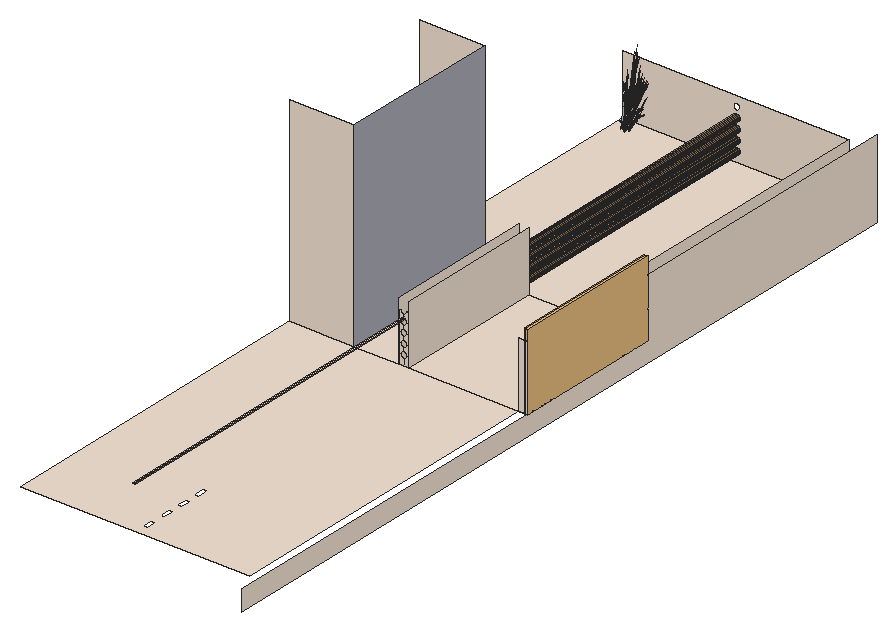
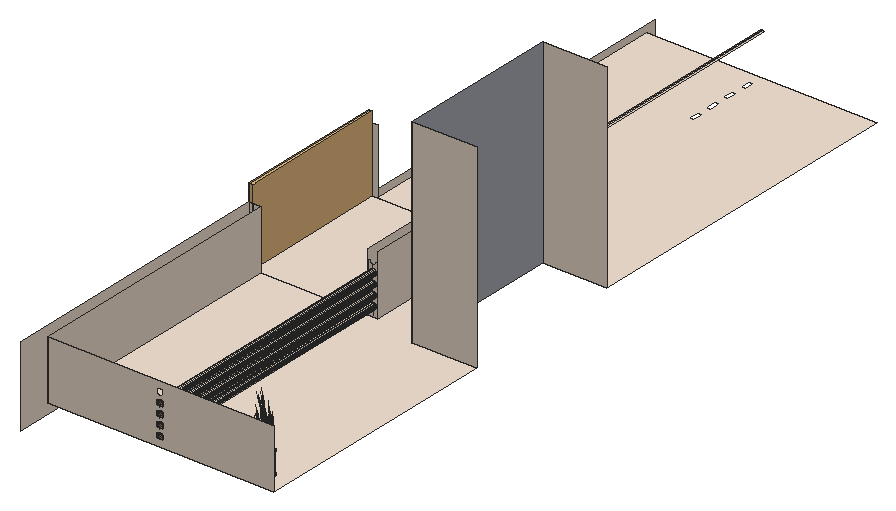
# SketchUp Ruby script. Lengths in inches.
U = 1.inch
M = Sketchup.active_model
def pt(a) = Geom::Point3d.new(a.map { |v| v * U })
def face(e, loops, mat)
  f = e.add_face(loops[0].map { |a| pt(a) })
  loops[1..].each { |l| e.add_face(l.map { |a| pt(a) }).erase! }
  f.material = f.back_material = mat if mat
  f
end
# faces: each face lists its corners as indices into pts; further lists are holes
def faces(e, pts, list, mat = nil) = list.each { |f| face(e, (f[0].is_a?(Array) ? f : [f]).map { |l| l.map { |i| pts[i] } }, mat) }
# xy, xz, yz: faces in a plane at the given z, y or x. An outline is a flat list of corners, or four numbers for a rectangle; further outlines are holes
def ring(l) = l.size == 4 ? [[l[0], l[1]], [l[2], l[1]], [l[2], l[3]], [l[0], l[3]]] : l.each_slice(2).to_a
def flat(e, list, mat, &to3) = list.each { |f| face(e, (f[0].is_a?(Array) ? f : [f]).map { |l| ring(l).map { |u, v| to3.(u, v) } }, mat) }
def xy(e, z, list, mat = nil) = flat(e, list, mat) { |x, y| [x, y, z] }
def xz(e, y, list, mat = nil) = flat(e, list, mat) { |x, z| [x, y, z] }
def yz(e, x, list, mat = nil) = flat(e, list, mat) { |y, z| [x, y, z] }
def lines(e, pts, list) = list.each { |a, b| e.add_line(pt(pts[a]), pt(pts[b])) }
# prism: a flat outline (further loops are holes) pulled along v
def prism(e, loops, v, mat = nil)
  f = face(e, loops, mat); d = Geom::Vector3d.new(v.map { |x| x * U })
  f.pushpull(f.normal.samedirection?(d) ? d.length : -d.length)
end
def box(e, o, s, mat = nil) = prism(e, [[o, [o[0] + s[0], o[1], o[2]], [o[0] + s[0], o[1] + s[1], o[2]], [o[0], o[1] + s[1], o[2]]]], [0, 0, s[2]], mat)
def at(x, y, z, deg = 0) = Geom::Transformation.translation(pt([x, y, z])) * Geom::Transformation.rotation(ORIGIN, Z_AXIS, deg.degrees)
def axes(o, x, y, z) = Geom::Transformation.new([*x, 0, *y, 0, *z, 0, *pt(o).to_a, 1])
def part(name) = M.definitions.add(name)
# library, detail: a bought-in or finely detailed component or shape, given as its bounding box
def library(name, o, s) = part(name).tap { |d| box(d.entities, o, s) }
def detail(e, o, s) = box(e.add_group.entities, o, s)
def put(e, d, t, mat = nil) = e.add_instance(d, t).tap { |i| i.material = mat if mat }
def group(e, t, mat = nil) = e.add_group.tap { |g| g.transformation = t; g.material = mat if mat }.entities
root = M.entities
M.materials.add("C01_Vanilla_Cream").color = [244, 228, 212]
M.materials.add("LightPink_Translucent").color = [144, 107, 117]
M.materials["LightPink_Translucent"].alpha = 0.75
M.materials.add("Marble_20_1K").color = [172, 173, 182]
M.materials.add("Wood_Floor_01_1K").color = [146, 111, 76]
c1 = part("blade")
p = [[2.15,0.21,22],[0,0.17,0],[0.09,0.45,0],[2.18,0.31,22],[2.29,0.31,22],[0.38,0.45,0],
  [2.48,0.24,33],[2.49,0.24,33],[2.48,0.22,33]]
faces(c1.entities,p,[[0,1,2,3],[4,5,2,3],[6,3,4,7],[8,0,3,6]])
c2 = part("seeds")
p = [[0.3,-0.1,1.38],[-0.01,-0.03,1.59],[-0.01,-0.03,0.03],[0.14,-0.07,-0.07],[0.29,-0.03,3],[0.15,0.01,3.11]]
faces(c2.entities,p,[[0,1,2,3],[1,0,4,5]],"LightPink_Translucent")
c3 = part("blade with seeds")
put(c3.entities,c1,at(0,0,0))
put(c3.entities,c2,axes([2.4,0.25,30.99],[1.5799,-0.05474,1.17369],[-0.12525,1.92788,0.29478],[-0.07173,-0.02425,1.56792]))
c4 = library("Modern+Gate+1",[0,0,0],[118.11,1.97,78.74])
xy(root,12,[[[288,12,426.72,216],[357,44.28,360,50.74],[357,18.46,360,24.91],[357,31.37,360,37.83],[357,57.2,360,63.65]],[326.85,216,354,216,354,306.76,424.7,306.76,424.7,468,288,468,288,314.71,326.85,314.71],[354,216,360,306.76],[360,216,432,306.76]],"C01_Vanilla_Cream")
xz(root,216,[[288,12,326.85,132],[354,12,357,12,357,16,356.48,16.07,356,16.27,355.59,16.59,355.27,17,355.07,17.48,355,18,354,18],[357,12,360,12,360,18,359,18,358.93,17.48,358.73,17,358.41,16.59,358,16.27,357.52,16.07,357,16],[426.72,12,432,51.56],[354,18,355,18,355.07,18.52,355.27,19,355.59,19.41,356,19.73,356.48,19.93,357,20,357,22,356.48,22.07,356,22.27,355.59,22.59,355.27,23,355.07,23.48,355,24,354,24],
  [359,18,360,18,360,24,359,24,358.93,23.48,358.73,23,358.41,22.59,358,22.27,357.52,22.07,357,22,357,20,357.52,19.93,358,19.73,358.41,19.41,358.73,19,358.93,18.52],[354,24,355,24,355.07,24.52,355.27,25,355.59,25.41,356,25.73,356.48,25.93,357,26,357,28,356.48,28.07,356,28.27,355.59,28.59,355.27,29,355.07,29.48,355,30,354,30],[359,24,360,24,360,30,359,30,358.93,29.48,358.73,29,358.41,28.59,358,28.27,357.52,28.07,357,28,357,26,357.52,25.93,358,25.73,358.41,25.41,358.73,25,358.93,24.52],[354,30,355,30,355.07,30.52,355.27,31,355.59,31.41,356,31.73,356.48,31.93,357,32,357,34,356.48,34.07,356,34.27,355.59,34.59,355.27,35,355.07,35.48,355,36,354,36],[359,30,360,30,360,36,359,36,358.93,35.48,358.73,35,358.41,34.59,358,34.27,357.52,34.07,357,34,357,32,357.52,31.93,358,31.73,358.41,31.41,358.73,31,358.93,30.52],
  [354,36,355,36,355.07,36.52,355.27,37,355.59,37.41,356,37.73,356.48,37.93,357,38,357,40,356.48,40.07,356,40.27,355.59,40.59,355.27,41,355.07,41.48,355,42,354,42],[359,36,360,36,360,42,359,42,358.93,41.48,358.73,41,358.41,40.59,358,40.27,357.52,40.07,357,40,357,38,357.52,37.93,358,37.73,358.41,37.41,358.73,37,358.93,36.52]],"C01_Vanilla_Cream")
xz(root,306.76,[[354,12,354,18,355,18,355.07,17.48,355.27,17,355.59,16.59,356,16.27,356.48,16.07,357,16,357,12],[357,12,357,16,357.52,16.07,358,16.27,358.41,16.59,358.73,17,358.93,17.48,359,18,360,18,360,12],[424.7,12,432,48],[354,18,354,24,355,24,355.07,23.48,355.27,23,355.59,22.59,356,22.27,356.48,22.07,357,22,357,20,356.48,19.93,356,19.73,355.59,19.41,355.27,19,355.07,18.52,355,18],[359,18,358.93,18.52,358.73,19,358.41,19.41,358,19.73,357.52,19.93,357,20,357,22,357.52,22.07,358,22.27,358.41,22.59,358.73,23,358.93,23.48,359,24,360,24,360,18],
  [354,24,354,30,355,30,355.07,29.48,355.27,29,355.59,28.59,356,28.27,356.48,28.07,357,28,357,26,356.48,25.93,356,25.73,355.59,25.41,355.27,25,355.07,24.52,355,24],[359,24,358.93,24.52,358.73,25,358.41,25.41,358,25.73,357.52,25.93,357,26,357,28,357.52,28.07,358,28.27,358.41,28.59,358.73,29,358.93,29.48,359,30,360,30,360,24],[354,30,354,36,355,36,355.07,35.48,355.27,35,355.59,34.59,356,34.27,356.48,34.07,357,34,357,32,356.48,31.93,356,31.73,355.59,31.41,355.27,31,355.07,30.52,355,30],[359,30,358.93,30.52,358.73,31,358.41,31.41,358,31.73,357.52,31.93,357,32,357,34,357.52,34.07,358,34.27,358.41,34.59,358.73,35,358.93,35.48,359,36,360,36,360,30],[354,36,354,42,355,42,355.07,41.48,355.27,41,355.59,40.59,356,40.27,356.48,40.07,357,40,357,38,356.48,37.93,356,37.73,355.59,37.41,355.27,37,355.07,36.52,355,36],
  [359,36,358.93,36.52,358.73,37,358.41,37.41,358,37.73,357.52,37.93,357,38,357,40,357.52,40.07,358,40.27,358.41,40.59,358.73,41,358.93,41.48,359,42,360,42,360,36]],"C01_Vanilla_Cream")
xz(root,314.71,[[288,12,326.85,132]],"C01_Vanilla_Cream")
xz(root,468,[[[288,12,424.7,48],[357,40,356.48,40.07,356,40.27,355.59,40.59,355.27,41,355.07,41.48,355,42,355.07,42.52,355.27,43,355.59,43.41,356,43.73,356.48,43.93,357,44,357.52,43.93,358,43.73,358.41,43.41,358.73,43,358.93,42.52,359,42,358.93,41.48,358.73,41,358.41,40.59,358,40.27,357.52,40.07],[357,34,356.48,34.07,356,34.27,355.59,34.59,355.27,35,355.07,35.48,355,36,355.07,36.52,355.27,37,355.59,37.41,356,37.73,356.48,37.93,357,38,357.52,37.93,358,37.73,358.41,37.41,358.73,37,358.93,36.52,359,36,358.93,35.48,358.73,35,358.41,34.59,358,34.27,357.52,34.07],[357,28,356.48,28.07,356,28.27,355.59,28.59,355.27,29,355.07,29.48,355,30,355.07,30.52,355.27,31,355.59,31.41,356,31.73,356.48,31.93,357,32,357.52,31.93,358,31.73,358.41,31.41,358.73,31,358.93,30.52,359,30,358.93,29.48,358.73,29,358.41,28.59,358,28.27,357.52,28.07],[357,22,356.48,22.07,356,22.27,355.59,22.59,355.27,23,355.07,23.48,355,24,355.07,24.52,355.27,25,355.59,25.41,356,25.73,356.48,25.93,357,26,357.52,25.93,358,25.73,358.41,25.41,358.73,25,358.93,24.52,359,24,358.93,23.48,358.73,23,358.41,22.59,358,22.27,357.52,22.07],[357,16,356.48,16.07,356,16.27,355.59,16.59,355.27,17,355.07,17.48,355,18,355.07,18.52,355.27,19,355.59,19.41,356,19.73,356.48,19.93,357,20,357.52,19.93,358,19.73,358.41,19.41,358.73,19,358.93,18.52,359,18,358.93,17.48,358.73,17,358.41,16.59,358,16.27,357.52,16.07]]],"C01_Vanilla_Cream")
yz(root,326.85,[[216,12,314.71,132]],"Marble_20_1K")
yz(root,354,[[216,12,306.76,48]],"C01_Vanilla_Cream")
yz(root,360,[[216,12,306.76,48]],"C01_Vanilla_Cream")
yz(root,424.7,[[306.76,12,468,48]],"C01_Vanilla_Cream")
yz(root,432,[[0,0,480,0,480,48,306.76,48,306.76,12,0,12]],"C01_Vanilla_Cream")
p = [[357,306.76,16],[356.48,306.76,16.07],[356.48,468,16.07],[357,468,16],[357.52,306.76,16.07],[357.52,468,16.07],
  [356,306.76,16.27],[356,468,16.27],[358,306.76,16.27],[358,468,16.27],[355.59,306.76,16.59],[355.59,468,16.59],
  [358.41,306.76,16.59],[358.41,468,16.59],[355.27,306.76,17],[355.27,468,17],[358.73,306.76,17],[358.73,468,17],
  [355.07,306.76,17.48],[355.07,468,17.48],[358.93,306.76,17.48],[358.93,468,17.48],[355,306.76,18],[355,468,18],
  [359,306.76,18],[359,468,18],[355.07,306.76,18.52],[355.07,468,18.52],[358.93,306.76,18.52],[358.93,468,18.52],
  [355.27,306.76,19],[355.27,468,19],[358.73,306.76,19],[358.73,468,19],[355.59,306.76,19.41],[355.59,468,19.41],
  [358.41,306.76,19.41],[358.41,468,19.41],[356,306.76,19.73],[356,468,19.73],[358,306.76,19.73],[358,468,19.73],
  [356.48,306.76,19.93],[356.48,468,19.93],[357.52,306.76,19.93],[357.52,468,19.93],[357,306.76,20],[357,468,20],
  [357,306.76,22],[356.48,306.76,22.07],[356.48,468,22.07],[357,468,22],[357.52,306.76,22.07],[357.52,468,22.07],
  [356,306.76,22.27],[356,468,22.27],[358,306.76,22.27],[358,468,22.27],[355.59,306.76,22.59],[355.59,468,22.59],
  [358.41,306.76,22.59],[358.41,468,22.59],[355.27,306.76,23],[355.27,468,23],[358.73,306.76,23],[358.73,468,23],
  [355.07,306.76,23.48],[355.07,468,23.48],[358.93,306.76,23.48],[358.93,468,23.48],[355,306.76,24],[355,468,24],
  [359,306.76,24],[359,468,24],[355.07,306.76,24.52],[355.07,468,24.52],[358.93,306.76,24.52],[358.93,468,24.52],
  [355.27,306.76,25],[355.27,468,25],[358.73,306.76,25],[358.73,468,25],[355.59,306.76,25.41],[355.59,468,25.41],
  [358.41,306.76,25.41],[358.41,468,25.41],[356,306.76,25.73],[356,468,25.73],[358,306.76,25.73],[358,468,25.73],
  [356.48,306.76,25.93],[356.48,468,25.93],[357.52,306.76,25.93],[357.52,468,25.93],[357,306.76,26],[357,468,26],
  [357,306.76,28],[356.48,306.76,28.07],[356.48,468,28.07],[357,468,28],[357.52,306.76,28.07],[357.52,468,28.07],
  [356,306.76,28.27],[356,468,28.27],[358,306.76,28.27],[358,468,28.27],[355.59,306.76,28.59],[355.59,468,28.59],
  [358.41,306.76,28.59],[358.41,468,28.59],[355.27,306.76,29],[355.27,468,29],[358.73,306.76,29],[358.73,468,29],
  [355.07,306.76,29.48],[355.07,468,29.48],[358.93,306.76,29.48],[358.93,468,29.48],[355,306.76,30],[355,468,30],
  [359,306.76,30],[359,468,30],[355.07,306.76,30.52],[355.07,468,30.52],[358.93,306.76,30.52],[358.93,468,30.52],
  [355.27,306.76,31],[355.27,468,31],[358.73,306.76,31],[358.73,468,31],[355.59,306.76,31.41],[355.59,468,31.41],
  [358.41,306.76,31.41],[358.41,468,31.41],[356,306.76,31.73],[356,468,31.73],[358,306.76,31.73],[358,468,31.73],
  [356.48,306.76,31.93],[356.48,468,31.93],[357.52,306.76,31.93],[357.52,468,31.93],[357,306.76,32],[357,468,32],
  [357,306.76,34],[356.48,306.76,34.07],[356.48,468,34.07],[357,468,34],[357.52,306.76,34.07],[357.52,468,34.07],
  [356,306.76,34.27],[356,468,34.27],[358,306.76,34.27],[358,468,34.27],[355.59,306.76,34.59],[355.59,468,34.59],
  [358.41,306.76,34.59],[358.41,468,34.59],[355.27,306.76,35],[355.27,468,35],[358.73,306.76,35],[358.73,468,35],
  [355.07,306.76,35.48],[355.07,468,35.48],[358.93,306.76,35.48],[358.93,468,35.48],[355,306.76,36],[355,468,36],
  [359,306.76,36],[359,468,36],[355.07,306.76,36.52],[355.07,468,36.52],[358.93,306.76,36.52],[358.93,468,36.52],
  [355.27,306.76,37],[355.27,468,37],[358.73,306.76,37],[358.73,468,37],[355.59,306.76,37.41],[355.59,468,37.41],
  [358.41,306.76,37.41],[358.41,468,37.41],[356,306.76,37.73],[356,468,37.73],[358,306.76,37.73],[358,468,37.73],
  [356.48,216,37.93],[356,216,37.73],[356,12,37.73],[356.48,12,37.93],[358,216,37.73],[357.52,216,37.93],
  [357.52,12,37.93],[358,12,37.73],[356.48,306.76,37.93],[356.48,468,37.93],[357.52,306.76,37.93],[357.52,468,37.93],
  [357,306.76,38],[357,468,38]]
faces(root,p,[[0,1,2,3],[1,6,7,2],[6,10,11,7],[10,14,15,11],[14,18,19,15],[18,22,23,19],[22,26,27,23],[26,30,31,27],
  [30,34,35,31],[34,38,39,35],[38,42,43,39],[42,46,47,43],[48,49,50,51],[49,54,55,50],[54,58,59,55],[58,62,63,59],
  [62,66,67,63],[66,70,71,67],[70,74,75,71],[74,78,79,75],[78,82,83,79],[82,86,87,83],[86,90,91,87],[90,94,95,91],
  [96,97,98,99],[97,102,103,98],[102,106,107,103],[106,110,111,107],[110,114,115,111],[114,118,119,115],[118,122,123,119],[122,126,127,123],
  [126,130,131,127],[130,134,135,131],[134,138,139,135],[138,142,143,139],[144,145,146,147],[145,150,151,146],[150,154,155,151],[154,158,159,155],
  [158,162,163,159],[162,166,167,163],[166,170,171,167],[170,174,175,171],[174,178,179,175],[178,182,183,179],[186,187,188,189],[182,194,195,183],
  [194,198,199,195]],"C01_Vanilla_Cream")
faces(root,p,[[4,0,3,5],[8,4,5,9],[12,8,9,13],[16,12,13,17],[20,16,17,21],[24,20,21,25],[28,24,25,29],[32,28,29,33],
  [36,32,33,37],[40,36,37,41],[44,40,41,45],[46,44,45,47],[52,48,51,53],[56,52,53,57],[60,56,57,61],[64,60,61,65],
  [68,64,65,69],[72,68,69,73],[76,72,73,77],[80,76,77,81],[84,80,81,85],[88,84,85,89],[92,88,89,93],[94,92,93,95],
  [100,96,99,101],[104,100,101,105],[108,104,105,109],[112,108,109,113],[116,112,113,117],[120,116,117,121],[124,120,121,125],[128,124,125,129],
  [132,128,129,133],[136,132,133,137],[140,136,137,141],[142,140,141,143],[148,144,147,149],[152,148,149,153],[156,152,153,157],[160,156,157,161],
  [164,160,161,165],[168,164,165,169],[172,168,169,173],[176,172,173,177],[180,176,177,181],[184,180,181,185],[190,191,192,193],[196,184,185,197],
  [198,196,197,199]],"Wood_Floor_01_1K")
put(root,c3,axes([298.36,456.53,15.55],[0.45752,0.02296,0.04823],[-0.01254,0.34663,0.37966],[0.04787,-0.13278,0.57892]))
put(root,c3,axes([298.31,459.73,14.07],[-0.31347,-0.14166,0.86145],[0.40476,-0.14393,0.63294],[0.10917,0.12192,0.18974]))
put(root,c3,axes([297.19,459.58,13.94],[0.00982,-0.16331,1.07251],[0.4695,-0.18242,-0.23066],[0.14493,0.19547,0.45856]))
put(root,c3,axes([298.82,455.96,15.54],[-0.00537,-0.09805,1.31208],[-0.45391,-0.28338,-0.2075],[0.07018,-0.17178,0.10523]))
put(root,c3,axes([296.63,457.26,13.54],[0.375,-0.3703,-0.46765],[0.46584,0.33578,-0.12274],[0.15027,-0.09237,1.03225]))
put(root,c3,axes([298.22,456.5,15.55],[0.39645,0.33614,0.36002],[-0.42102,0.2899,0.29685],[0.07313,-0.15771,0.74497]))
put(root,c3,axes([298.28,456.93,13.52],[0.13078,0.42928,-0.23233],[-0.51941,0.1219,0.23233],[0.10471,0.0495,1.0423]))
put(root,c3,axes([299.25,458.33,13.78],[0.69617,0,0],[0,0.55062,-0.38706],[0,0.12541,1.22783]))
put(root,c3,axes([297,457.62,14],[0.56211,-0.32708,-0.21822],[0.3738,0.46216,-0.37502],[0.13869,0.04694,1.19781]))
put(root,c3,axes([298.36,460.375,14],[-0.35702,-0.01545,0.78795],[0.23577,-0.32816,0.43504],[0.14104,0.11659,0.61808]))
put(root,c3,axes([298.67,457.56,15.79],[-0.48462,0.07041,0.2656],[-0.12797,-0.4025,-0.3429],[0.13888,-0.10811,0.65611]))
put(root,c3,axes([297.28,456.4375,14.91],[-0.10366,0.16934,1.28532],[-0.43488,-0.35044,0.10393],[0.19618,-0.21841,0.54946]))
put(root,c3,axes([297.21,460.13,15.78],[0.33176,-0.4217,-0.0912],[0.48044,0.24295,-0.50621],[0.16701,0.11914,0.76918]))
put(root,c3,axes([295.59,457.33,13.2],[-0.548,0.19724,0.96696],[-0.17442,-0.56594,0.37572],[0.3365,0.00941,1.09981]))
put(root,c3,axes([298.93,457.6,15.78],[-0.515,-0.27165,-0.0912],[0.2967,-0.3934,-0.50621],[0.1455,-0.13675,0.76918]))
put(root,c3,axes([297.6,459.92,15.51],[0.54938,-0.11711,-0.38324],[0.0961,0.44351,-0.29685],[0.14756,0.1271,0.7333]))
put(root,c3,axes([298.1,456.45,13.78],[0.34808,-0.49367,0],[0.58235,0.27531,-0.38706],[0.13264,0.0627,1.22783]))
put(root,c3,axes([298.6875,456.24,13.12],[-0.08333,-0.03881,1.32257],[-0.21404,-0.4336,-0.20205],[0.14439,-0.11767,0.22528]))
put(root,c3,axes([298.23,459.39,15.79],[-0.31678,-0.30846,0.2656],[0.36171,-0.29199,-0.3429],[0.18378,0.04443,0.65611]))
put(root,c3,axes([298.42,456.75,13.51],[0.52105,0.24633,-0.37238],[-0.31144,0.44171,0],[0.11867,0.0561,1.18128]))
put(root,c3,axes([298.52,459.67,15.55],[-0.02803,0.37463,0.04823],[-0.42332,-0.01027,0.37966],[0.16216,0.0392,0.57892]))
put(root,c3,axes([298.4,460.26,13.12],[0.04056,-0.07113,1.32257],[0.51066,-0.20948,-0.20205],[0.15482,0.10842,0.22528]))
put(root,c3,axes([298.56,459.55,15.55],[-0.41051,0.32462,0.36002],[-0.35404,-0.34474,0.29685],[0.1926,0.05988,0.74497]))
put(root,c3,axes([298.67,457.28,15.51],[-0.14302,-0.44985,-0.38324],[0.54163,-0.07869,-0.29685],[0.15522,-0.12083,0.7333]))
put(root,c3,axes([299.625,459.6,14.95],[-0.10656,-0.41414,-0.02619],[0.50364,-0.09521,-0.11874],[0.10517,0.02626,0.39164]))
put(root,c3,axes([298.75,458.53,15.79],[-0.46269,-0.13744,0.2656],[0.13495,-0.40096,-0.3429],[0.18628,-0.03677,0.65611]))
put(root,c3,axes([297.66,457.69,13.54],[0.57914,0.08077,-0.46765],[-0.12221,0.49823,-0.12274],[0.17283,0.06037,1.03225]))
put(root,c3,axes([300.13,457.99,13.7],[-0.34516,-0.31503,-0.04866],[0.37803,-0.28865,-0.22062],[0.10711,-0.02032,0.72768]))
put(root,c3,axes([299.34,456.38,14.07],[-0.18544,0.25079,0.86145],[-0.15939,-0.33694,0.63294],[0.15316,-0.08443,0.18974]))
put(root,c3,axes([299.11,457.5,15.55],[0.3822,0.20719,0.04823],[-0.22252,0.29505,0.37966],[0.12254,-0.09539,0.57892]))
put(root,c3,axes([299.01,457.41,15.55],[0.13808,0.45342,0.36002],[-0.54163,0.07869,0.29685],[0.15963,-0.10664,0.74497]))
put(root,c3,axes([297.54,458.76,14.91],[-0.2068,-0.08488,1.28532],[0.42797,-0.35609,0.10393],[0.26673,0.16064,0.54946]))
put(root,c3,axes([300.19,457.48,15.53],[-0.07272,-0.00374,1.33037],[-0.30197,-0.40092,-0.12571],[0.12127,-0.13182,0.23543]))
put(root,c3,axes([299.07,457.33,15.39],[0.48462,-0.07041,-0.2656],[0.12797,0.4025,0.3429],[0.13888,-0.10811,0.65611]))
put(root,c3,axes([298.68,457.46,15.74],[0.29081,-0.38873,-0.53284],[0.5096,0.27626,0.0643],[0.17364,-0.14084,0.75375]))
put(root,c3,axes([299.17,458.65,15.55],[0.20448,0.33592,0.04823],[-0.37288,0.16442,0.37966],[0.16437,-0.03244,0.57892]))
put(root,c3,axes([298.68,459.55,15.39],[0.31678,0.30846,-0.2656],[-0.36171,0.29199,0.3429],[0.18378,0.04443,0.65611]))
put(root,c3,axes([298.32,459.59,15.78],[0.02981,-0.50103,-0.0912],[0.56442,0.01369,-0.50621],[0.21738,0.0348,0.76918]))
put(root,c3,axes([298.95,458.66,15.78],[-0.28012,-0.44611,-0.0912],[0.49717,-0.21923,-0.50621],[0.20951,-0.05886,0.76918]))
put(root,c3,axes([299.13,458.53,15.55],[-0.15729,0.44921,0.36002],[-0.51712,-0.15361,0.29685],[0.20336,-0.027,0.74497]))
put(root,c3,axes([298.81,459.29,15.54],[0.11943,-0.00833,1.31208],[0.32759,-0.38275,-0.2075],[0.21244,0.05052,0.10523]))
put(root,c3,axes([298.92,458.28,15.51],[0.15083,-0.44814,-0.38324],[0.51712,0.15361,-0.29685],[0.2082,-0.04109,0.7333]))
put(root,c3,axes([300.22,458.5625,14.07],[-0.34399,0.08133,0.86145],[0.16192,-0.33614,0.63294],[0.18249,0.023,0.18974]))
put(root,c3,axes([299.11,457.1,13.94],[-0.19889,-0.01459,1.07251],[-0.20376,-0.39145,-0.23066],[0.24434,-0.11074,0.45856]))
put(root,c3,axes([299.24,458.48,15.39],[0.46269,0.13744,-0.2656],[-0.13495,0.40096,0.3429],[0.18628,-0.03677,0.65611]))
put(root,c3,axes([298.35,459.35,15.74],[0.55654,0.01186,-0.53284],[-0.03738,0.49951,0.0643],[0.23578,0.05271,0.75375]))
put(root,c3,axes([299.47,458.4,13.49],[-0.35858,0.05912,1.06187],[-0.05708,-0.47061,0.06078],[0.25115,-0.07123,0.60425]))
put(root,c3,axes([299.87,458.1,13.12],[-0.0291,-0.0748,1.32257],[0.20181,-0.43752,-0.20205],[0.20357,-0.00629,0.22528]))
put(root,c3,axes([300.0625,459.99,15.53],[-0.05034,-0.04313,1.33037],[0.11012,-0.46232,-0.12571],[0.1983,-0.02954,0.23543]))
put(root,c3,axes([297.98,457.99,14.91],[-0.23093,0.01116,1.28532],[0.15319,-0.4836,0.10393],[0.32909,0.02991,0.54946]))
put(root,c3,axes([298.82,458.44,15.74],[0.48922,-0.21758,-0.53284],[0.27264,0.44789,0.0643],[0.23638,-0.05088,0.75375]))
put(root,c3,axes([300.47,457.96,15.54],[0.07726,-0.07504,1.31208],[-0.09888,-0.46032,-0.2075],[0.19384,-0.08728,0.10523]))
put(root,c3,axes([299.58,459.1,13.94],[-0.13408,-0.12117,1.07251],[0.17446,-0.40083,-0.23066],[0.27128,0.0543,0.45856]))
put(root,c4,axes([430.03,306.76,12],[0,-0.76843,0],[1,0,0],[0,0,0.5852]))
